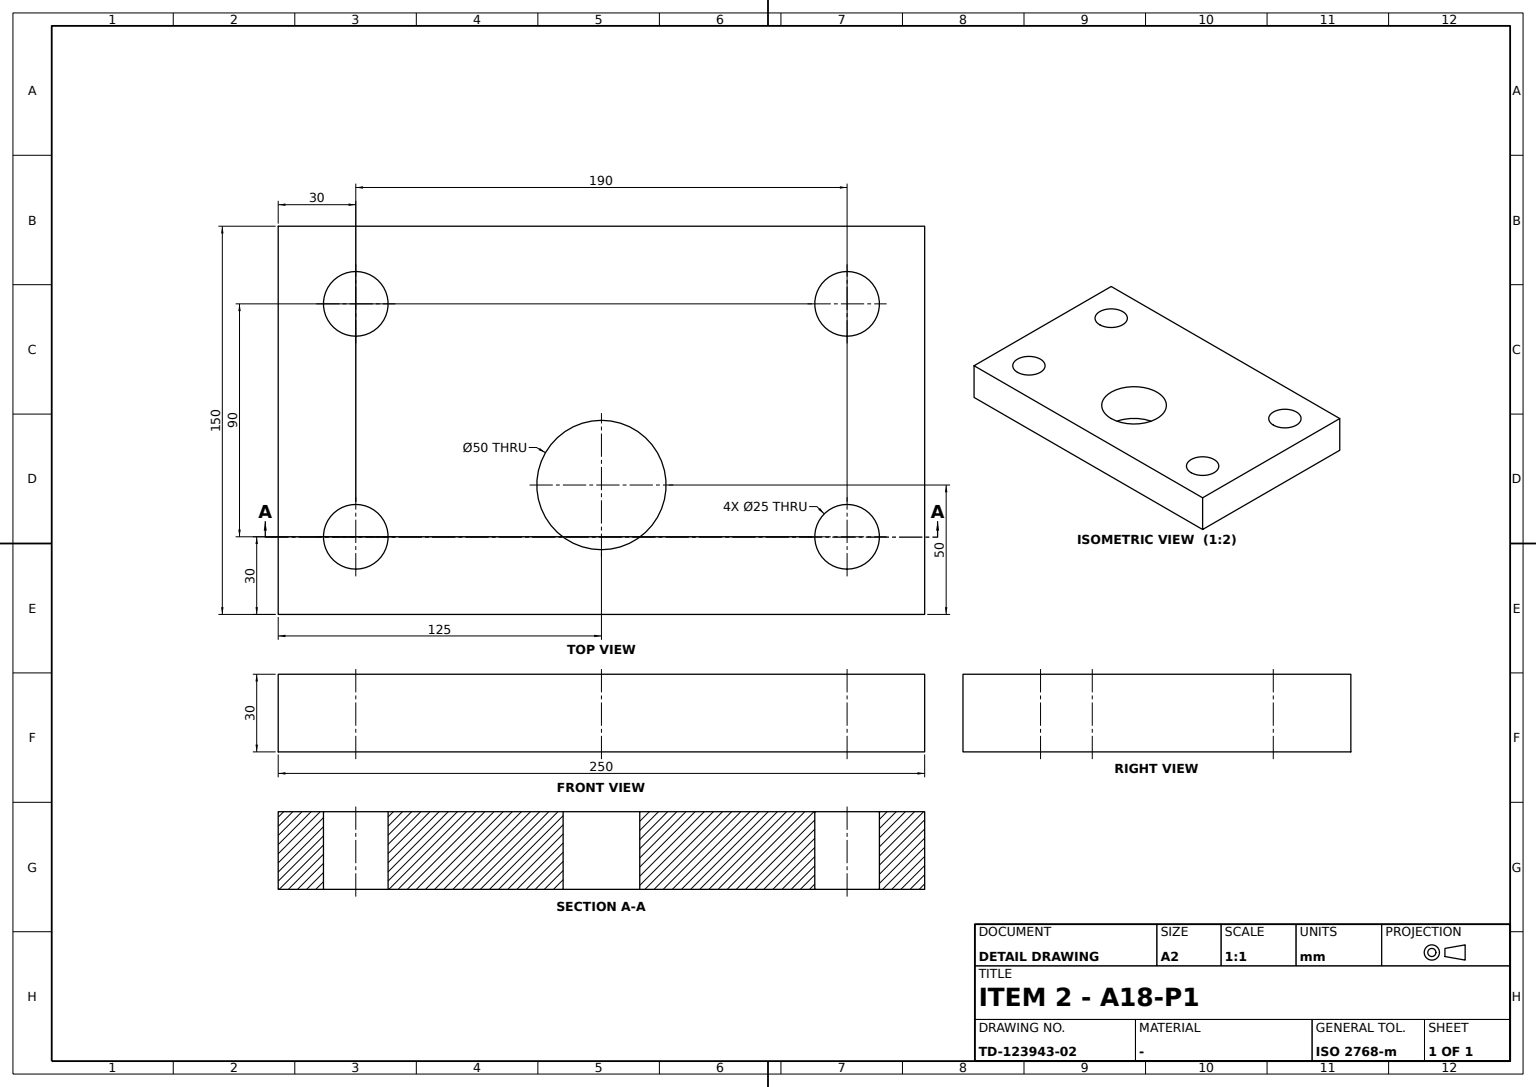
ISO-10303-21;
HEADER;
FILE_DESCRIPTION((''),'2;1');
FILE_NAME('','',(''),(''),'','','');
FILE_SCHEMA(('AUTOMOTIVE_DESIGN'));
ENDSEC;
DATA;
#1=APPLICATION_CONTEXT('');
#2=PRODUCT_CONTEXT('',#1,'mechanical');
#3=PRODUCT('','','',(#2));
#4=PRODUCT_DEFINITION_FORMATION('','',#3);
#5=PRODUCT_DEFINITION_CONTEXT('',#1,'design');
#6=PRODUCT_DEFINITION('','',#4,#5);
#7=PRODUCT_DEFINITION_SHAPE('','',#6);
#8=(LENGTH_UNIT()NAMED_UNIT(*)SI_UNIT(.MILLI.,.METRE.));
#9=(NAMED_UNIT(*)PLANE_ANGLE_UNIT()SI_UNIT($,.RADIAN.));
#10=(NAMED_UNIT(*)SI_UNIT($,.STERADIAN.)SOLID_ANGLE_UNIT());
#11=UNCERTAINTY_MEASURE_WITH_UNIT(LENGTH_MEASURE(0.005),#8,'distance_accuracy_value','');
#12=(GEOMETRIC_REPRESENTATION_CONTEXT(3)GLOBAL_UNCERTAINTY_ASSIGNED_CONTEXT((#11))GLOBAL_UNIT_ASSIGNED_CONTEXT((#8,#9,#10))REPRESENTATION_CONTEXT('',''));
#13=CARTESIAN_POINT('',(57.5,95.,-15.));
#14=VERTEX_POINT('',#13);
#15=CARTESIAN_POINT('',(45.,95.,-15.));
#16=DIRECTION('',(0.,0.,1.));
#17=DIRECTION('',(1.,0.,0.));
#18=AXIS2_PLACEMENT_3D('',#15,#16,#17);
#19=CIRCLE('',#18,12.5);
#20=EDGE_CURVE('',#14,#14,#19,.F.);
#21=ORIENTED_EDGE('',*,*,#20,.T.);
#22=EDGE_LOOP('',(#21));
#23=FACE_BOUND('',#22,.T.);
#24=CARTESIAN_POINT('',(57.5,95.,15.));
#25=VERTEX_POINT('',#24);
#26=CARTESIAN_POINT('',(45.,95.,15.));
#27=AXIS2_PLACEMENT_3D('',#26,#16,#17);
#28=CIRCLE('',#27,12.5);
#29=EDGE_CURVE('',#25,#25,#28,.T.);
#30=ORIENTED_EDGE('',*,*,#29,.T.);
#31=EDGE_LOOP('',(#30));
#32=FACE_BOUND('',#31,.T.);
#33=CARTESIAN_POINT('',(45.,95.,14.9));
#34=DIRECTION('',(0.,0.,-1.));
#35=AXIS2_PLACEMENT_3D('',#33,#34,#17);
#36=CYLINDRICAL_SURFACE('',#35,12.5);
#37=ADVANCED_FACE('',(#23,#32),#36,.F.);
#38=CARTESIAN_POINT('',(-32.5,-95.,-15.));
#39=VERTEX_POINT('',#38);
#40=CARTESIAN_POINT('',(-45.,-95.,-15.));
#41=AXIS2_PLACEMENT_3D('',#40,#16,#17);
#42=CIRCLE('',#41,12.5);
#43=EDGE_CURVE('',#39,#39,#42,.F.);
#44=ORIENTED_EDGE('',*,*,#43,.T.);
#45=EDGE_LOOP('',(#44));
#46=FACE_BOUND('',#45,.T.);
#47=CARTESIAN_POINT('',(-32.5,-95.,15.));
#48=VERTEX_POINT('',#47);
#49=CARTESIAN_POINT('',(-45.,-95.,15.));
#50=AXIS2_PLACEMENT_3D('',#49,#16,#17);
#51=CIRCLE('',#50,12.5);
#52=EDGE_CURVE('',#48,#48,#51,.T.);
#53=ORIENTED_EDGE('',*,*,#52,.T.);
#54=EDGE_LOOP('',(#53));
#55=FACE_BOUND('',#54,.T.);
#56=CARTESIAN_POINT('',(-45.,-95.,14.9));
#57=AXIS2_PLACEMENT_3D('',#56,#34,#17);
#58=CYLINDRICAL_SURFACE('',#57,12.5);
#59=ADVANCED_FACE('',(#46,#55),#58,.F.);
#60=CARTESIAN_POINT('',(-75.,-125.,-15.));
#61=VERTEX_POINT('',#60);
#62=CARTESIAN_POINT('',(-75.,-125.,15.));
#63=VERTEX_POINT('',#62);
#64=CARTESIAN_POINT('',(-75.,-125.,0.));
#65=VECTOR('',#16,1000.);
#66=LINE('',#64,#65);
#67=EDGE_CURVE('',#61,#63,#66,.T.);
#68=ORIENTED_EDGE('',*,*,#67,.T.);
#69=CARTESIAN_POINT('',(-75.,125.,15.));
#70=VERTEX_POINT('',#69);
#71=CARTESIAN_POINT('',(-75.,0.,15.));
#72=DIRECTION('',(0.,1.,0.));
#73=VECTOR('',#72,1000.);
#74=LINE('',#71,#73);
#75=EDGE_CURVE('',#63,#70,#74,.T.);
#76=ORIENTED_EDGE('',*,*,#75,.T.);
#77=CARTESIAN_POINT('',(-75.,125.,-15.));
#78=VERTEX_POINT('',#77);
#79=CARTESIAN_POINT('',(-75.,125.,0.));
#80=LINE('',#79,#65);
#81=EDGE_CURVE('',#78,#70,#80,.T.);
#82=ORIENTED_EDGE('',*,*,#81,.F.);
#83=CARTESIAN_POINT('',(-75.,0.,-15.));
#84=LINE('',#83,#73);
#85=EDGE_CURVE('',#61,#78,#84,.T.);
#86=ORIENTED_EDGE('',*,*,#85,.F.);
#87=EDGE_LOOP('',(#68,#76,#82,#86));
#88=FACE_BOUND('',#87,.T.);
#89=AXIS2_PLACEMENT_3D('',#64,#17,#72);
#90=PLANE('',#89);
#91=ADVANCED_FACE('',(#88),#90,.F.);
#92=CARTESIAN_POINT('',(50.,0.,-15.));
#93=VERTEX_POINT('',#92);
#94=CARTESIAN_POINT('',(25.,0.,-15.));
#95=AXIS2_PLACEMENT_3D('',#94,#16,#17);
#96=CIRCLE('',#95,25.);
#97=EDGE_CURVE('',#93,#93,#96,.T.);
#98=ORIENTED_EDGE('',*,*,#97,.F.);
#99=EDGE_LOOP('',(#98));
#100=FACE_BOUND('',#99,.T.);
#101=CARTESIAN_POINT('',(50.,0.,15.));
#102=VERTEX_POINT('',#101);
#103=CARTESIAN_POINT('',(25.,0.,15.));
#104=AXIS2_PLACEMENT_3D('',#103,#16,#17);
#105=CIRCLE('',#104,25.);
#106=EDGE_CURVE('',#102,#102,#105,.T.);
#107=ORIENTED_EDGE('',*,*,#106,.T.);
#108=EDGE_LOOP('',(#107));
#109=FACE_BOUND('',#108,.T.);
#110=CARTESIAN_POINT('',(25.,0.,0.));
#111=AXIS2_PLACEMENT_3D('',#110,#16,#72);
#112=CYLINDRICAL_SURFACE('',#111,25.);
#113=ADVANCED_FACE('',(#100,#109),#112,.F.);
#114=CARTESIAN_POINT('',(-32.5,95.,15.));
#115=VERTEX_POINT('',#114);
#116=CARTESIAN_POINT('',(-45.,95.,15.));
#117=AXIS2_PLACEMENT_3D('',#116,#16,#17);
#118=CIRCLE('',#117,12.5);
#119=EDGE_CURVE('',#115,#115,#118,.T.);
#120=ORIENTED_EDGE('',*,*,#119,.T.);
#121=EDGE_LOOP('',(#120));
#122=FACE_BOUND('',#121,.T.);
#123=CARTESIAN_POINT('',(-32.5,95.,-15.));
#124=VERTEX_POINT('',#123);
#125=CARTESIAN_POINT('',(-45.,95.,-15.));
#126=AXIS2_PLACEMENT_3D('',#125,#16,#17);
#127=CIRCLE('',#126,12.5);
#128=EDGE_CURVE('',#124,#124,#127,.F.);
#129=ORIENTED_EDGE('',*,*,#128,.T.);
#130=EDGE_LOOP('',(#129));
#131=FACE_BOUND('',#130,.T.);
#132=CARTESIAN_POINT('',(-45.,95.,14.9));
#133=AXIS2_PLACEMENT_3D('',#132,#34,#17);
#134=CYLINDRICAL_SURFACE('',#133,12.5);
#135=ADVANCED_FACE('',(#122,#131),#134,.F.);
#136=CARTESIAN_POINT('',(75.,125.,-15.));
#137=VERTEX_POINT('',#136);
#138=CARTESIAN_POINT('',(75.,-125.,-15.));
#139=VERTEX_POINT('',#138);
#140=CARTESIAN_POINT('',(75.,0.,-15.));
#141=DIRECTION('',(0.,-1.,0.));
#142=VECTOR('',#141,1000.);
#143=LINE('',#140,#142);
#144=EDGE_CURVE('',#137,#139,#143,.T.);
#145=ORIENTED_EDGE('',*,*,#144,.F.);
#146=CARTESIAN_POINT('',(75.,125.,15.));
#147=VERTEX_POINT('',#146);
#148=CARTESIAN_POINT('',(75.,125.,0.));
#149=LINE('',#148,#65);
#150=EDGE_CURVE('',#137,#147,#149,.T.);
#151=ORIENTED_EDGE('',*,*,#150,.T.);
#152=CARTESIAN_POINT('',(75.,-125.,15.));
#153=VERTEX_POINT('',#152);
#154=CARTESIAN_POINT('',(75.,0.,15.));
#155=LINE('',#154,#142);
#156=EDGE_CURVE('',#147,#153,#155,.T.);
#157=ORIENTED_EDGE('',*,*,#156,.T.);
#158=CARTESIAN_POINT('',(75.,-125.,0.));
#159=LINE('',#158,#65);
#160=EDGE_CURVE('',#139,#153,#159,.T.);
#161=ORIENTED_EDGE('',*,*,#160,.F.);
#162=EDGE_LOOP('',(#145,#151,#157,#161));
#163=FACE_BOUND('',#162,.T.);
#164=DIRECTION('',(-1.,0.,0.));
#165=AXIS2_PLACEMENT_3D('',#148,#164,#141);
#166=PLANE('',#165);
#167=ADVANCED_FACE('',(#163),#166,.F.);
#168=ORIENTED_EDGE('',*,*,#43,.F.);
#169=EDGE_LOOP('',(#168));
#170=FACE_BOUND('',#169,.T.);
#171=ORIENTED_EDGE('',*,*,#128,.F.);
#172=EDGE_LOOP('',(#171));
#173=FACE_BOUND('',#172,.T.);
#174=ORIENTED_EDGE('',*,*,#97,.T.);
#175=EDGE_LOOP('',(#174));
#176=FACE_BOUND('',#175,.T.);
#177=ORIENTED_EDGE('',*,*,#20,.F.);
#178=EDGE_LOOP('',(#177));
#179=FACE_BOUND('',#178,.T.);
#180=CARTESIAN_POINT('',(0.,-125.,-15.));
#181=VECTOR('',#164,1000.);
#182=LINE('',#180,#181);
#183=EDGE_CURVE('',#139,#61,#182,.T.);
#184=ORIENTED_EDGE('',*,*,#183,.T.);
#185=ORIENTED_EDGE('',*,*,#85,.T.);
#186=CARTESIAN_POINT('',(0.,125.,-15.));
#187=VECTOR('',#17,1000.);
#188=LINE('',#186,#187);
#189=EDGE_CURVE('',#78,#137,#188,.T.);
#190=ORIENTED_EDGE('',*,*,#189,.T.);
#191=ORIENTED_EDGE('',*,*,#144,.T.);
#192=EDGE_LOOP('',(#184,#185,#190,#191));
#193=FACE_BOUND('',#192,.T.);
#194=CARTESIAN_POINT('',(57.5,-95.,-15.));
#195=VERTEX_POINT('',#194);
#196=CARTESIAN_POINT('',(45.,-95.,-15.));
#197=AXIS2_PLACEMENT_3D('',#196,#16,#17);
#198=CIRCLE('',#197,12.5);
#199=EDGE_CURVE('',#195,#195,#198,.F.);
#200=ORIENTED_EDGE('',*,*,#199,.F.);
#201=EDGE_LOOP('',(#200));
#202=FACE_BOUND('',#201,.T.);
#203=CARTESIAN_POINT('',(0.,0.,-15.));
#204=AXIS2_PLACEMENT_3D('',#203,#16,#72);
#205=PLANE('',#204);
#206=ADVANCED_FACE('',(#170,#173,#176,#179,#193,#202),#205,.F.);
#207=ORIENTED_EDGE('',*,*,#160,.T.);
#208=CARTESIAN_POINT('',(0.,-125.,15.));
#209=LINE('',#208,#181);
#210=EDGE_CURVE('',#153,#63,#209,.T.);
#211=ORIENTED_EDGE('',*,*,#210,.T.);
#212=ORIENTED_EDGE('',*,*,#67,.F.);
#213=ORIENTED_EDGE('',*,*,#183,.F.);
#214=EDGE_LOOP('',(#207,#211,#212,#213));
#215=FACE_BOUND('',#214,.T.);
#216=AXIS2_PLACEMENT_3D('',#158,#72,#164);
#217=PLANE('',#216);
#218=ADVANCED_FACE('',(#215),#217,.F.);
#219=ORIENTED_EDGE('',*,*,#199,.T.);
#220=EDGE_LOOP('',(#219));
#221=FACE_BOUND('',#220,.T.);
#222=CARTESIAN_POINT('',(57.5,-95.,15.));
#223=VERTEX_POINT('',#222);
#224=CARTESIAN_POINT('',(45.,-95.,15.));
#225=AXIS2_PLACEMENT_3D('',#224,#16,#17);
#226=CIRCLE('',#225,12.5);
#227=EDGE_CURVE('',#223,#223,#226,.T.);
#228=ORIENTED_EDGE('',*,*,#227,.T.);
#229=EDGE_LOOP('',(#228));
#230=FACE_BOUND('',#229,.T.);
#231=CARTESIAN_POINT('',(45.,-95.,14.9));
#232=AXIS2_PLACEMENT_3D('',#231,#34,#17);
#233=CYLINDRICAL_SURFACE('',#232,12.5);
#234=ADVANCED_FACE('',(#221,#230),#233,.F.);
#235=ORIENTED_EDGE('',*,*,#81,.T.);
#236=CARTESIAN_POINT('',(0.,125.,15.));
#237=LINE('',#236,#187);
#238=EDGE_CURVE('',#70,#147,#237,.T.);
#239=ORIENTED_EDGE('',*,*,#238,.T.);
#240=ORIENTED_EDGE('',*,*,#150,.F.);
#241=ORIENTED_EDGE('',*,*,#189,.F.);
#242=EDGE_LOOP('',(#235,#239,#240,#241));
#243=FACE_BOUND('',#242,.T.);
#244=AXIS2_PLACEMENT_3D('',#79,#141,#17);
#245=PLANE('',#244);
#246=ADVANCED_FACE('',(#243),#245,.F.);
#247=ORIENTED_EDGE('',*,*,#119,.F.);
#248=EDGE_LOOP('',(#247));
#249=FACE_BOUND('',#248,.T.);
#250=ORIENTED_EDGE('',*,*,#156,.F.);
#251=ORIENTED_EDGE('',*,*,#238,.F.);
#252=ORIENTED_EDGE('',*,*,#75,.F.);
#253=ORIENTED_EDGE('',*,*,#210,.F.);
#254=EDGE_LOOP('',(#250,#251,#252,#253));
#255=FACE_BOUND('',#254,.T.);
#256=ORIENTED_EDGE('',*,*,#227,.F.);
#257=EDGE_LOOP('',(#256));
#258=FACE_BOUND('',#257,.T.);
#259=ORIENTED_EDGE('',*,*,#106,.F.);
#260=EDGE_LOOP('',(#259));
#261=FACE_BOUND('',#260,.T.);
#262=ORIENTED_EDGE('',*,*,#29,.F.);
#263=EDGE_LOOP('',(#262));
#264=FACE_BOUND('',#263,.T.);
#265=ORIENTED_EDGE('',*,*,#52,.F.);
#266=EDGE_LOOP('',(#265));
#267=FACE_BOUND('',#266,.T.);
#268=CARTESIAN_POINT('',(0.,0.,15.));
#269=AXIS2_PLACEMENT_3D('',#268,#16,#72);
#270=PLANE('',#269);
#271=ADVANCED_FACE('',(#249,#255,#258,#261,#264,#267),#270,.T.);
#272=CLOSED_SHELL('',(#37,#59,#91,#113,#135,#167,#206,#218,#234,#246,#271));
#273=MANIFOLD_SOLID_BREP('',#272);
#274=ADVANCED_BREP_SHAPE_REPRESENTATION('',(#273),#12);
#275=SHAPE_DEFINITION_REPRESENTATION(#7,#274);
ENDSEC;
END-ISO-10303-21;
